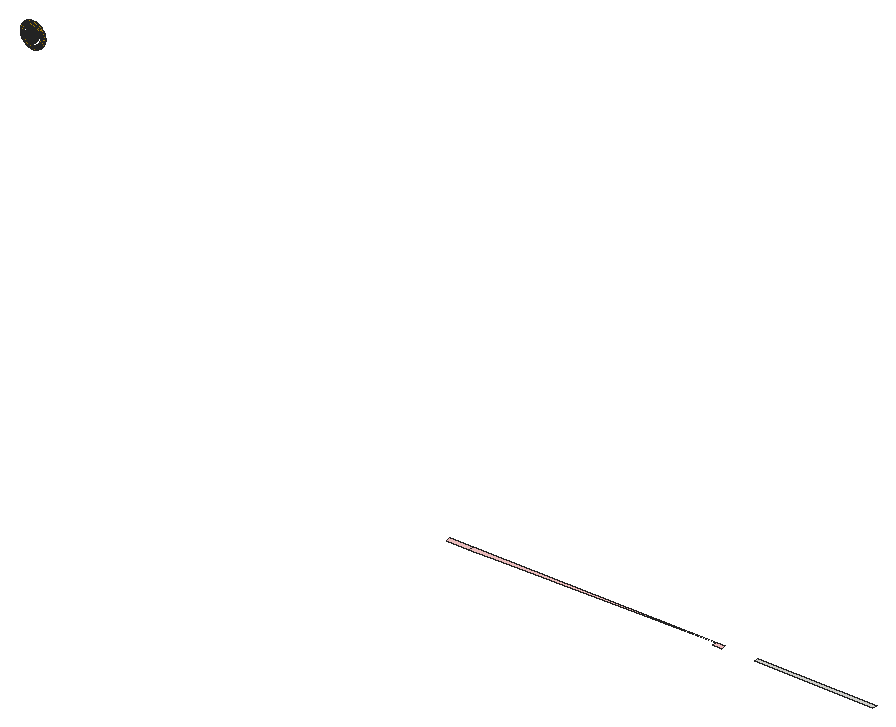
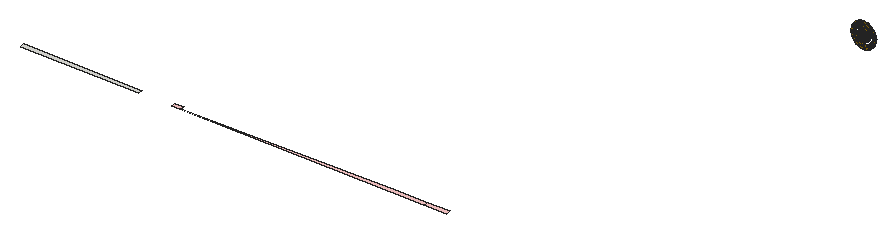
# SketchUp Ruby script. Lengths in inches.
U = 1.inch
M = Sketchup.active_model
def pt(a) = Geom::Point3d.new(a.map { |v| v * U })
def face(e, loops, mat)
  f = e.add_face(loops[0].map { |a| pt(a) })
  loops[1..].each { |l| e.add_face(l.map { |a| pt(a) }).erase! }
  f.material = f.back_material = mat if mat
  f
end
# faces: each face lists its corners as indices into pts; further lists are holes
def faces(e, pts, list, mat = nil) = list.each { |f| face(e, (f[0].is_a?(Array) ? f : [f]).map { |l| l.map { |i| pts[i] } }, mat) }
# xy, xz, yz: faces in a plane at the given z, y or x. An outline is a flat list of corners, or four numbers for a rectangle; further outlines are holes
def ring(l) = l.size == 4 ? [[l[0], l[1]], [l[2], l[1]], [l[2], l[3]], [l[0], l[3]]] : l.each_slice(2).to_a
def flat(e, list, mat, &to3) = list.each { |f| face(e, (f[0].is_a?(Array) ? f : [f]).map { |l| ring(l).map { |u, v| to3.(u, v) } }, mat) }
def xy(e, z, list, mat = nil) = flat(e, list, mat) { |x, y| [x, y, z] }
def xz(e, y, list, mat = nil) = flat(e, list, mat) { |x, z| [x, y, z] }
def yz(e, x, list, mat = nil) = flat(e, list, mat) { |y, z| [x, y, z] }
def lines(e, pts, list) = list.each { |a, b| e.add_line(pt(pts[a]), pt(pts[b])) }
# prism: a flat outline (further loops are holes) pulled along v
def prism(e, loops, v, mat = nil)
  f = face(e, loops, mat); d = Geom::Vector3d.new(v.map { |x| x * U })
  f.pushpull(f.normal.samedirection?(d) ? d.length : -d.length)
end
def box(e, o, s, mat = nil) = prism(e, [[o, [o[0] + s[0], o[1], o[2]], [o[0] + s[0], o[1] + s[1], o[2]], [o[0], o[1] + s[1], o[2]]]], [0, 0, s[2]], mat)
def at(x, y, z, deg = 0) = Geom::Transformation.translation(pt([x, y, z])) * Geom::Transformation.rotation(ORIGIN, Z_AXIS, deg.degrees)
def axes(o, x, y, z) = Geom::Transformation.new([*x, 0, *y, 0, *z, 0, *pt(o).to_a, 1])
def part(name) = M.definitions.add(name)
# library, detail: a bought-in or finely detailed component or shape, given as its bounding box
def library(name, o, s) = part(name).tap { |d| box(d.entities, o, s) }
def detail(e, o, s) = box(e.add_group.entities, o, s)
def put(e, d, t, mat = nil) = e.add_instance(d, t).tap { |i| i.material = mat if mat }
def group(e, t, mat = nil) = e.add_group.tap { |g| g.transformation = t; g.material = mat if mat }.entities
root = M.entities
M.materials.add("[Color A01]").color = [255, 204, 204]
M.materials.add("[Color D06]").color = [204, 153, 0]
xy(root,46.28,[[240,753.18,261.625,754.01]])
xy(root,46.28,[[183.68,753.18,187.82,753.18,187.75,754.01,183.68,754.01],[187.82,753.18,187.75,754.01,232.4375,754.01,193.19,753.18],[232.4375,753.18,234,754.01]],"[Color A01]")
xz(root,753.58,[[106.625,102.81,106.7,102.9,106.41,103.17,106.31,103.04],[106.7,102.9,106.79,102.99,106.52,103.28,106.41,103.17],[108.4,102.9,108.69,103.17,108.58,103.28,108.32,102.99],[106.79,102.99,106.88,103.0625,106.65,103.38,106.52,103.28],[108.32,102.99,108.58,103.28,108.45,103.38,108.22,103.0625],
  [106.88,103.0625,106.98,103.13,106.78,103.47,106.65,103.38],[108.22,103.0625,108.45,103.38,108.32,103.47,108.12,103.13],[106.98,103.13,107.09,103.18,106.93,103.54,106.78,103.47],[108.12,103.13,108.32,103.47,108.18,103.54,108.02,103.18],[107.09,103.18,107.2,103.23,107.08,103.6,106.93,103.54],
  [108.02,103.18,108.18,103.54,108.03,103.6,107.9,103.23],[107.2,103.23,107.3125,103.26,107.23,103.64,107.08,103.6],[107.9,103.23,108.03,103.6,107.87,103.64,107.79,103.26],[107.3125,103.26,107.43,103.28,107.39,103.67,107.23,103.64],[107.79,103.26,107.87,103.64,107.71,103.67,107.67,103.28],
  [107.43,103.28,107.55,103.28,107.55,103.68,107.39,103.67],[107.55,103.28,107.67,103.28,107.71,103.67,107.55,103.68]],"[Color D06]")
p = [[107.31,753.75,99.84],[107.35,753.64,100.22],[107.15,753.64,100.25],[107.07,753.75,99.88],[107.55,753.75,99.83],[107.55,753.64,100.21],
  [107.79,753.75,99.84],[107.75,753.64,100.22],[108.03,753.75,99.88],[107.95,753.64,100.25],[106.84,753.75,99.94],[106.96,753.64,100.31],
  [106.77,753.64,100.38],[106.61,753.75,100.03],[108.26,753.75,99.94],[108.15,753.64,100.31],[108.49,753.75,100.03],[108.33,753.64,100.38],
  [106.59,753.64,100.47],[106.4,753.75,100.14],[108.7,753.75,100.14],[108.51,753.64,100.47],[106.42,753.64,100.58],[106.19,753.75,100.27],
  [108.91,753.75,100.27],[108.68,753.64,100.58],[107.39,753.58,100.61],[107.23,753.58,100.63],[107.55,753.58,100.6],[107.71,753.58,100.61],
  [107.87,753.58,100.63],[106.26,753.64,100.71],[106.01,753.75,100.42],[107.08,753.58,100.68],[106.93,753.58,100.73],[108.03,753.58,100.68],
  [108.18,753.58,100.73],[109.09,753.75,100.42],[108.84,753.64,100.71],[106.12,753.64,100.85],[105.84,753.75,100.59],[106.78,753.58,100.81],
  [108.32,753.58,100.81],[109.26,753.75,100.59],[108.98,753.64,100.85],[106.65,753.58,100.89],[108.45,753.58,100.89],[105.99,753.64,101.01],
  [105.68,753.75,100.78],[106.52,753.58,101],[108.58,753.58,101],[109.42,753.75,100.78],[109.11,753.64,101.01],[106.41,753.58,101.11],
  [108.69,753.58,101.11],[105.88,753.64,101.17],[105.55,753.75,100.98],[106.31,753.58,101.23],[108.79,753.58,101.23],[109.55,753.75,100.98],
  [109.22,753.64,101.17],[105.79,753.64,101.35],[105.44,753.75,101.2],[106.22,753.58,101.37],[107.3125,753.58,101.02],[107.39,753.62,101.4],
  [107.32,753.62,101.42],[107.2,753.58,101.05],[107.43,753.58,101],[107.47,753.62,101.39],[107.55,753.58,100.99],[107.55,753.62,101.39],
  [107.67,753.58,101],[107.63,753.62,101.39],[107.79,753.58,101.02],[107.71,753.62,101.4],[107.9,753.58,101.05],[107.78,753.62,101.42],
  [108.88,753.58,101.37],[109.66,753.75,101.2],[109.3125,753.64,101.35],[106.98,753.58,101.15],[107.17,753.62,101.49],[107.11,753.62,101.53],
  [106.88,753.58,101.21],[107.09,753.58,101.09],[107.24,753.62,101.45],[108.02,753.58,101.09],[107.86,753.62,101.45],[108.12,753.58,101.15],
  [107.93,753.62,101.49],[108.22,753.58,101.21],[107.99,753.62,101.53],[105.72,753.64,101.54],[105.36,753.75,101.43],[106.15,753.58,101.51],
  [107.05,753.62,101.58],[106.79,753.58,101.29],[108.32,753.58,101.29],[108.05,753.62,101.58],[108.95,753.58,101.51],[109.74,753.75,101.43],
  [109.38,753.64,101.54],[106.99,753.62,101.64],[106.7,753.58,101.375],[108.4,753.58,101.375],[108.11,753.62,101.64],[105.67,753.64,101.74],
  [105.29,753.75,101.66],[106.09,753.58,101.66],[106.94,753.62,101.7],[106.625,753.58,101.47],[107.4375,753.71,101.79],[107.4,753.71,101.8],
  [107.47,753.71,101.78],[107.51,753.71,101.77],[107.55,753.71,101.77],[107.59,753.71,101.77],[107.63,753.71,101.78],[107.66,753.71,101.79],
  [107.7,753.71,101.8],[108.48,753.58,101.47],[108.16,753.62,101.7],[109.01,753.58,101.66],[109.81,753.75,101.66],[109.44,753.64,101.74],
  [106.05,753.58,101.82],[106.9,753.62,101.76],[106.56,753.58,101.57],[107.33,753.71,101.84],[107.3,753.71,101.86],[107.37,753.71,101.82],
  [107.73,753.71,101.82],[107.77,753.71,101.84],[107.8,753.71,101.86],[108.54,753.58,101.57],[108.2,753.62,101.76],[109.05,753.58,101.82],
  [106.86,753.62,101.83],[106.51,753.58,101.67],[107.28,753.71,101.89],[107.25,753.71,101.92],[107.82,753.71,101.89],[107.85,753.71,101.92],
  [108.59,753.58,101.67],[108.24,753.62,101.83],[105.63,753.64,101.9375],[105.26,753.75,101.9],[106.02,753.58,101.98],[106.84,753.62,101.91],
  [106.46,753.58,101.78],[107.23,753.71,101.95],[107.87,753.71,101.95],[108.64,753.58,101.78],[108.27,753.62,101.91],[109.47,753.64,101.9375],
  [109.08,753.58,101.98],[109.84,753.75,101.9],[106.82,753.62,101.98],[106.43,753.58,101.9],[107.21,753.71,101.99],[107.2,753.71,102.02],
  [107.89,753.71,101.99],[107.9,753.71,102.02],[108.67,753.58,101.9],[108.29,753.62,101.98],[107.55,753.85,102.14],[105.625,753.64,102.14],
  [105.24,753.75,102.14],[106.01,753.58,102.14],[106.8,753.62,102.06],[106.41,753.58,102.02],[107.19,753.71,102.0625],[107.91,753.71,102.0625],
  [108.6875,753.58,102.02],[108.3,753.62,102.06],[109.48,753.64,102.14],[109.09,753.58,102.14],[109.86,753.75,102.14],[106.8,753.62,102.14],
  [106.41,753.58,102.14],[107.18,753.71,102.1],[107.92,753.71,102.1],[108.69,753.58,102.14],[108.3,753.62,102.14],[105.63,753.64,102.34],
  [105.26,753.75,102.38],[106.02,753.58,102.3],[106.8,753.62,102.22],[106.41,753.58,102.26],[107.18,753.71,102.14],[107.18,753.71,102.18],
  [107.92,753.71,102.14],[108.3,753.62,102.22],[107.92,753.71,102.18],[108.6875,753.58,102.26],[109.47,753.64,102.34],[109.08,753.58,102.3],
  [109.84,753.75,102.38],[107.59,753.71,102.5],[107.63,753.71,102.5],[107.66,753.71,102.49],[107.55,753.71,102.51],[107.8,753.71,102.41],
  [107.82,753.71,102.38],[107.7,753.71,102.47],[107.73,753.71,102.46],[106.82,753.62,102.29],[106.43,753.58,102.375],[107.19,753.71,102.21],
  [107.2,753.71,102.25],[106.84,753.62,102.37],[108.29,753.62,102.29],[107.91,753.71,102.21],[108.27,753.62,102.37],[107.9,753.71,102.25],
  [108.67,753.58,102.375],[105.67,753.64,102.54],[105.29,753.75,102.62],[106.05,753.58,102.46],[106.46,753.58,102.49],[107.21,753.71,102.29],
  [106.86,753.62,102.44],[107.23,753.71,102.32],[106.9,753.62,102.51],[107.25,753.71,102.35],[106.94,753.62,102.58],[108.16,753.62,102.58],
  [107.85,753.71,102.35],[107.87,753.71,102.32],[108.2,753.62,102.51],[108.24,753.62,102.44],[107.89,753.71,102.29],[108.64,753.58,102.49],
  [109.44,753.64,102.54],[109.05,753.58,102.46],[109.81,753.75,102.62],[106.51,753.58,102.6],[106.56,753.58,102.71],[107.28,753.71,102.38],
  [106.99,753.62,102.64],[107.3,753.71,102.41],[107.05,753.62,102.7],[107.33,753.71,102.4375],[107.11,753.62,102.75],[107.37,753.71,102.46],
  [107.17,753.62,102.79],[107.93,753.62,102.79],[107.77,753.71,102.4375],[107.99,753.62,102.75],[108.11,753.62,102.64],[108.05,753.62,102.7],
  [108.59,753.58,102.6],[108.54,753.58,102.71],[105.72,753.64,102.73],[105.36,753.75,102.85],[106.09,753.58,102.61],[106.625,753.58,102.81],
  [107.4,753.71,102.47],[107.24,753.62,102.82],[107.4375,753.71,102.49],[107.32,753.62,102.85],[107.47,753.71,102.5],[107.39,753.62,102.875],
  [107.51,753.71,102.5],[107.47,753.62,102.89],[107.55,753.62,102.89],[107.71,753.62,102.875],[107.78,753.62,102.85],[107.63,753.62,102.89],
  [107.86,753.62,102.82],[108.48,753.58,102.81],[109.38,753.64,102.73],[109.01,753.58,102.61],[109.74,753.75,102.85],[106.15,753.58,102.76],
  [105.79,753.64,102.92],[106.7,753.58,102.9],[106.79,753.58,102.99],[108.4,753.58,102.9],[108.32,753.58,102.99],[109.3125,753.64,102.92],
  [108.95,753.58,102.76],[105.44,753.75,103.08],[106.88,753.58,103.0625],[106.98,753.58,103.13],[108.12,753.58,103.13],[108.22,753.58,103.0625],
  [109.66,753.75,103.08],[106.22,753.58,102.91],[105.88,753.64,103.1],[107.09,753.58,103.18],[107.2,753.58,103.23],[107.9,753.58,103.23],
  [108.02,753.58,103.18],[109.22,753.64,103.1],[108.88,753.58,102.91],[105.55,753.75,103.29],[106.31,753.58,103.04],[105.99,753.64,103.27],
  [107.3125,753.58,103.26],[107.43,753.58,103.28],[107.55,753.58,103.28],[107.67,753.58,103.28],[107.79,753.58,103.26],[109.11,753.64,103.27],
  [108.79,753.58,103.04],[109.55,753.75,103.29],[106.41,753.58,103.17],[106.12,753.64,103.43],[108.98,753.64,103.43],[108.69,753.58,103.17],
  [105.68,753.75,103.49],[109.42,753.75,103.49],[106.52,753.58,103.28],[106.26,753.64,103.57],[108.84,753.64,103.57],[108.58,753.58,103.28],
  [105.84,753.75,103.68],[106.65,753.58,103.38],[106.42,753.64,103.7],[108.68,753.64,103.7],[108.45,753.58,103.38],[109.26,753.75,103.68],
  [106.01,753.75,103.85],[106.78,753.58,103.47],[106.59,753.64,103.81],[108.51,753.64,103.81],[108.32,753.58,103.47],[109.09,753.75,103.85],
  [106.93,753.58,103.54],[106.77,753.64,103.9],[107.08,753.58,103.6],[106.96,753.64,103.97],[108.15,753.64,103.97],[108.03,753.58,103.6],
  [108.18,753.58,103.54],[108.33,753.64,103.9],[106.19,753.75,104],[107.23,753.58,103.64],[107.15,753.64,104.02],[107.39,753.58,103.67],
  [107.35,753.64,104.05],[107.75,753.64,104.05],[107.71,753.58,103.67],[107.87,753.58,103.64],[107.95,753.64,104.02],[108.91,753.75,104],
  [106.4,753.75,104.14],[107.55,753.58,103.68],[107.55,753.64,104.06],[108.7,753.75,104.14],[106.61,753.75,104.25],[108.49,753.75,104.25],
  [106.84,753.75,104.33],[108.26,753.75,104.33],[107.07,753.75,104.39],[107.31,753.75,104.43],[107.79,753.75,104.43],[108.03,753.75,104.39],
  [107.55,753.75,104.44]]
faces(root,p,[[0,1,2,3],[4,5,1,0],[6,7,5,4],[8,9,7,6],[10,11,12,13],[3,2,11,10],[14,15,9,8],[16,17,15,14],
  [13,12,18,19],[20,21,17,16],[19,18,22,23],[24,25,21,20],[1,26,27,2],[5,28,26,1],[7,29,28,5],[9,30,29,7],
  [23,22,31,32],[11,33,34,12],[2,27,33,11],[15,35,30,9],[17,36,35,15],[37,38,25,24],[32,31,39,40],[12,34,41,18],
  [21,42,36,17],[43,44,38,37],[18,41,45,22],[25,46,42,21],[40,39,47,48],[22,45,49,31],[38,50,46,25],[51,52,44,43],
  [31,49,53,39],[44,54,50,38],[48,47,55,56],[39,53,57,47],[52,58,54,44],[59,60,52,51],[56,55,61,62],[47,57,63,55],
  [64,65,66,67],[68,69,65,64],[70,71,69,68],[72,73,71,70],[74,75,73,72],[76,77,75,74],[60,78,58,52],[79,80,60,59],
  [81,82,83,84],[85,86,82,81],[67,66,86,85],[87,88,77,76],[89,90,88,87],[91,92,90,89],[62,61,93,94],[55,63,95,61],
  [84,83,96,97],[98,99,92,91],[80,100,78,60],[101,102,80,79],[97,96,103,104],[105,106,99,98],[94,93,107,108],[61,95,109,93],
  [104,103,110,111],[66,112,113,86],[65,114,112,66],[69,115,114,65],[71,116,115,69],[73,117,116,71],[75,118,117,73],[77,119,118,75],
  [88,120,119,77],[121,122,106,105],[102,123,100,80],[124,125,102,101],[93,109,126,107],[111,110,127,128],[83,129,130,96],[82,131,129,83],
  [86,113,131,82],[90,132,120,88],[92,133,132,90],[99,134,133,92],[135,136,122,121],[125,137,123,102],[128,127,138,139],[103,140,141,110],
  [96,130,140,103],[106,142,134,99],[122,143,142,106],[144,145,136,135],[108,107,146,147],[107,126,148,146],[139,138,149,150],[110,141,151,127],
  [136,152,143,122],[153,154,145,144],[155,156,137,125],[157,155,125,124],[150,149,158,159],[138,160,161,149],[127,151,160,138],[145,162,152,136],
  [154,163,162,145],[164,165,154,153],[131,166,129],[129,166,130],[114,166,112],[112,166,113],[113,166,131],[116,166,115],
  [115,166,114],[117,166,116],[118,166,117],[119,166,118],[120,166,119],[132,166,120],[133,166,132],[134,166,133],
  [147,146,167,168],[146,148,169,167],[159,158,170,171],[149,161,172,158],[165,173,163,154],[174,175,165,164],[176,177,156,155],[178,176,155,157],
  [141,166,151],[130,166,140],[140,166,141],[142,166,134],[143,166,142],[152,166,143],[171,170,179,180],[158,172,181,170],
  [175,182,173,165],[183,184,175,174],[151,166,160],[160,166,161],[161,166,172],[162,166,152],[163,166,162],[173,166,163],
  [168,167,185,186],[167,169,187,185],[180,179,188,189],[170,181,190,179],[179,190,191,188],[184,192,182,175],[193,194,192,184],[195,193,184,183],
  [196,197,177,176],[198,196,176,178],[172,166,181],[181,166,190],[182,166,173],[192,166,182],[199,166,200],[200,166,201],
  [202,166,199],[203,166,204],[201,166,205],[205,166,206],[189,188,207,208],[188,191,209,207],[207,209,210,211],[212,213,194,193],
  [214,215,213,212],[216,212,193,195],[186,185,217,218],[185,187,219,217],[208,207,211,220],[211,210,221,222],[222,221,223,224],[224,223,225,226],
  [227,228,229,230],[231,232,215,214],[230,229,232,231],[233,214,212,216],[234,235,197,196],[236,234,196,198],[220,211,222,237],[237,222,224,238],
  [226,225,239,240],[240,239,241,242],[242,241,243,244],[244,243,245,246],[247,206,248,249],[250,204,228,227],[251,203,204,250],[249,248,203,251],
  [252,231,214,233],[253,230,231,252],[218,217,254,255],[217,219,256,254],[238,224,226,257],[246,245,258,259],[259,258,260,261],[261,260,262,263],
  [263,262,264,265],[265,264,202,266],[267,200,201,268],[269,199,200,267],[266,202,199,269],[270,205,206,247],[268,201,205,270],[271,227,230,253],
  [272,273,235,234],[274,272,234,236],[254,256,275,276],[257,226,240,277],[277,240,242,278],[279,250,227,271],[280,251,250,279],[281,282,273,272],
  [255,254,276,283],[278,242,244,284],[284,244,246,285],[286,247,249,287],[287,249,251,280],[288,281,272,274],[276,275,289,290],[285,246,259,291],
  [291,259,261,292],[293,268,270,294],[294,270,247,286],[295,296,282,281],[283,276,290,297],[290,289,298,299],[292,261,263,300],[300,263,265,301],
  [301,265,266,302],[303,269,267,304],[302,266,269,303],[304,267,268,293],[305,306,296,295],[307,295,281,288],[299,298,308,309],[310,311,306,305],
  [297,290,299,312],[313,305,295,307],[309,308,314,315],[316,317,311,310],[312,299,309,318],[315,314,319,320],[321,322,317,316],[323,310,305,313],
  [318,309,315,324],[320,319,325,326],[327,328,322,321],[329,316,310,323],[326,325,330,331],[331,330,332,333],[334,335,336,337],[337,336,328,327],
  [324,315,320,338],[333,332,339,340],[340,339,341,342],[343,344,345,346],[346,345,335,334],[347,321,316,329],[338,320,326,348],[342,341,349,350],
  [350,349,344,343],[351,327,321,347],[348,326,331,352],[353,337,327,351],[352,331,333,354],[355,334,337,353],[354,333,340,356],[356,340,342,357],
  [358,343,346,359],[359,346,334,355],[357,342,350,360],[360,350,343,358]],"[Color D06]")
